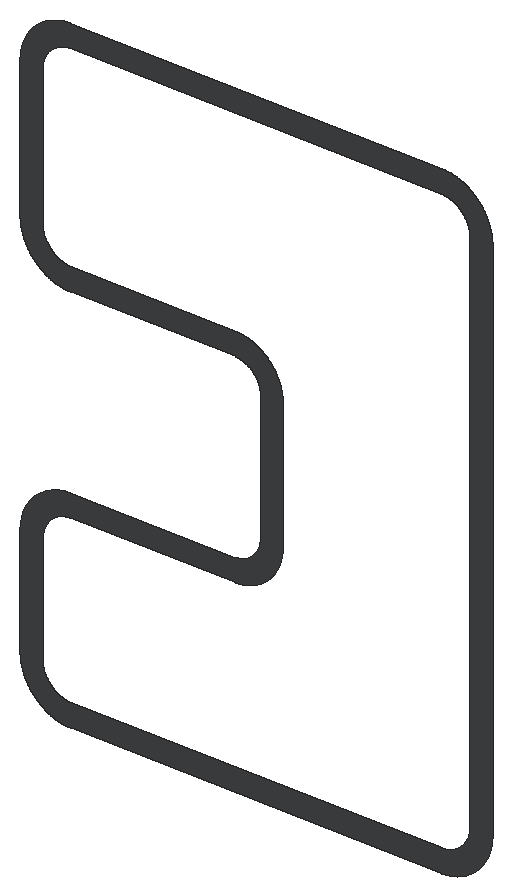
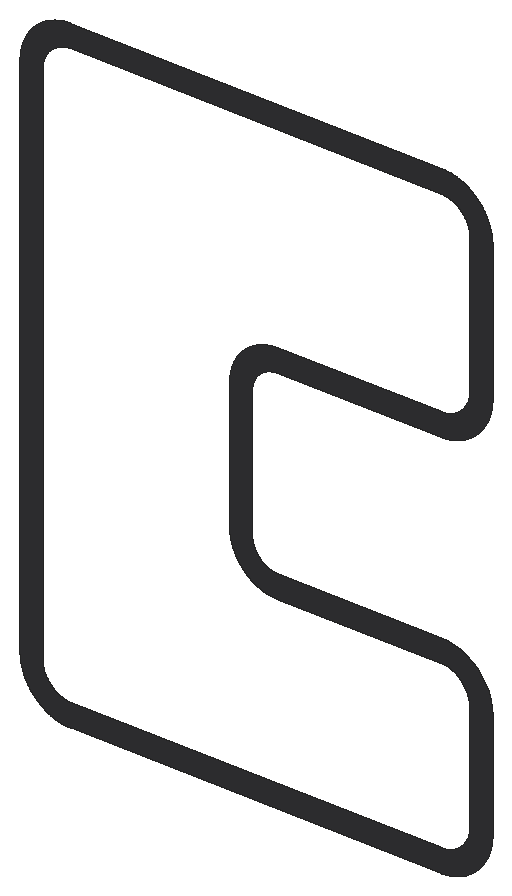
# SketchUp Ruby script. Lengths in inches.
U = 1.inch
M = Sketchup.active_model
def pt(a) = Geom::Point3d.new(a.map { |v| v * U })
def face(e, loops, mat)
  f = e.add_face(loops[0].map { |a| pt(a) })
  loops[1..].each { |l| e.add_face(l.map { |a| pt(a) }).erase! }
  f.material = f.back_material = mat if mat
  f
end
# faces: each face lists its corners as indices into pts; further lists are holes
def faces(e, pts, list, mat = nil) = list.each { |f| face(e, (f[0].is_a?(Array) ? f : [f]).map { |l| l.map { |i| pts[i] } }, mat) }
# xy, xz, yz: faces in a plane at the given z, y or x. An outline is a flat list of corners, or four numbers for a rectangle; further outlines are holes
def ring(l) = l.size == 4 ? [[l[0], l[1]], [l[2], l[1]], [l[2], l[3]], [l[0], l[3]]] : l.each_slice(2).to_a
def flat(e, list, mat, &to3) = list.each { |f| face(e, (f[0].is_a?(Array) ? f : [f]).map { |l| ring(l).map { |u, v| to3.(u, v) } }, mat) }
def xy(e, z, list, mat = nil) = flat(e, list, mat) { |x, y| [x, y, z] }
def xz(e, y, list, mat = nil) = flat(e, list, mat) { |x, z| [x, y, z] }
def yz(e, x, list, mat = nil) = flat(e, list, mat) { |y, z| [x, y, z] }
def lines(e, pts, list) = list.each { |a, b| e.add_line(pt(pts[a]), pt(pts[b])) }
# prism: a flat outline (further loops are holes) pulled along v
def prism(e, loops, v, mat = nil)
  f = face(e, loops, mat); d = Geom::Vector3d.new(v.map { |x| x * U })
  f.pushpull(f.normal.samedirection?(d) ? d.length : -d.length)
end
def box(e, o, s, mat = nil) = prism(e, [[o, [o[0] + s[0], o[1], o[2]], [o[0] + s[0], o[1] + s[1], o[2]], [o[0], o[1] + s[1], o[2]]]], [0, 0, s[2]], mat)
def at(x, y, z, deg = 0) = Geom::Transformation.translation(pt([x, y, z])) * Geom::Transformation.rotation(ORIGIN, Z_AXIS, deg.degrees)
def axes(o, x, y, z) = Geom::Transformation.new([*x, 0, *y, 0, *z, 0, *pt(o).to_a, 1])
def part(name) = M.definitions.add(name)
# library, detail: a bought-in or finely detailed component or shape, given as its bounding box
def library(name, o, s) = part(name).tap { |d| box(d.entities, o, s) }
def detail(e, o, s) = box(e.add_group.entities, o, s)
def put(e, d, t, mat = nil) = e.add_instance(d, t).tap { |i| i.material = mat if mat }
def group(e, t, mat = nil) = e.add_group.tap { |g| g.transformation = t; g.material = mat if mat }.entities
root = M.entities
M.materials.add("1432 AP 8245 TAR ROAD").color = [71, 72, 75]
xz(root,95.37,[[[278.72,155.79,537.28,155.79,537.57,155.8,537.85,155.8,538.41,155.82,538.7,155.83,538.98,155.85,539.26,155.86,539.82,155.9,540.11,155.93,540.39,155.95,541.23,156.04,541.51,156.08,541.79,156.11,542.35,156.19,542.63,156.24,542.91,156.28,543.1875,156.33,543.47,156.38,543.75,156.43,544.02,156.48,544.58,156.6,544.85,156.66,545.13,156.72,545.4,156.79,545.68,156.85,545.95,156.92,546.23,156.99,546.5,157.07,546.77,157.14,547.31,157.3,547.59,157.38,547.86,157.47,548.125,157.55,548.39,157.64,548.66,157.73,548.93,157.83,549.19,157.92,549.73,158.12,550.25,158.32,550.51,158.43,550.78,158.53,551.3,158.75,551.56,158.87,551.81,158.98,552.33,159.22,552.58,159.34,552.84,159.46,553.34,159.72,553.6,159.85,553.85,159.98,554.09,160.11,554.34,160.25,554.59,160.38,554.84,160.52,555.08,160.66,555.33,160.81,555.57,160.95,556.53,161.55,556.76,161.7,557.24,162.02,557.93,162.5,558.16,162.67,558.39,162.83,558.62,163,558.84,163.17,559.06,163.35,559.29,163.52,559.51,163.7,559.95,164.05,560.16,164.23,560.38,164.42,560.59,164.6,560.81,164.79,561.23,165.17,561.4375,165.36,561.64,165.55,561.85,165.74,562.05,165.94,562.26,166.14,562.46,166.34,562.65,166.54,563.05,166.94,563.24,167.15,563.4375,167.36,563.625,167.5625,563.82,167.77,564,167.98,564.19,168.2,564.375,168.41,564.56,168.63,564.74,168.84,564.92,169.0625,565.1,169.28,565.27,169.5,565.45,169.73,565.62,169.95,565.79,170.18,565.96,170.4,566.29,170.86,566.45,171.09,566.62,171.32,566.77,171.56,566.93,171.79,567.09,172.03,567.24,172.26,567.4,172.5,567.7,172.98,567.84,173.22,567.99,173.47,568.13,173.71,568.27,173.96,568.41,174.2,568.55,174.45,568.68,174.7,568.82,174.95,569.08,175.45,569.2,175.7,569.33,175.95,569.45,176.21,569.57,176.46,569.69,176.72,569.8125,176.98,569.93,177.24,570.04,177.49,570.15,177.75,570.26,178.02,570.37,178.28,570.47,178.54,570.58,178.8,570.68,179.07,570.77,179.33,570.87,179.6,570.97,179.86,571.24,180.67,571.32,180.9375,571.41,181.21,571.65,182.02,571.72,182.29,571.8,182.57,571.87,182.84,571.9375,183.11,572.01,183.39,572.07,183.66,572.13,183.9375,572.19,184.22,572.25,184.49,572.31,184.77,572.36,185.05,572.41,185.32,572.56,186.16,572.72,187.28,572.75,187.5625,572.78,187.84,572.8125,188.12,572.84,188.4,572.87,188.6875,572.89,188.97,572.93,189.53,572.95,189.8125,572.96,190.1,572.99,190.94,573,191.23,573,561.36,572.98,561.92,572.97,562.21,572.95,562.77,572.91,563.33,572.89,563.62,572.87,563.9,572.84,564.18,572.8125,564.46,572.78,564.74,572.72,565.3,572.56,566.42,572.31,567.82,572.25,568.09,572.13,568.65,572.07,568.92,572.01,569.2,571.9375,569.47,571.8,570.02,571.72,570.29,571.65,570.5625,571.57,570.84,571.41,571.38,571.32,571.65,571.24,571.92,571.15,572.19,571.06,572.45,570.97,572.72,570.87,572.99,570.77,573.25,570.68,573.52,570.58,573.78,570.47,574.04,570.37,574.31,569.93,575.35,569.8125,575.61,569.69,575.86,569.57,576.12,569.33,576.63,569.2,576.88,569.08,577.14,568.82,577.64,568.68,577.89,568.55,578.14,568.41,578.38,568.27,578.63,567.99,579.12,567.84,579.36,567.7,579.6,567.4,580.08,567.24,580.32,567.09,580.56,566.93,580.79,566.77,581.03,566.62,581.26,566.45,581.49,566.29,581.72,565.96,582.18,565.79,582.41,565.62,582.63,565.45,582.86,565.27,583.08,565.1,583.3,564.56,583.96,564.375,584.17,564.19,584.39,564,584.6,563.82,584.8125,563.625,585.02,563.4375,585.23,563.24,585.4375,563.05,585.64,562.85,585.84,562.65,586.05,562.46,586.25,562.26,586.45,562.05,586.64,561.85,586.84,561.64,587.03,561.4375,587.23,561.23,587.42,560.81,587.8,560.59,587.98,560.38,588.17,560.16,588.35,559.95,588.53,559.51,588.89,559.29,589.0625,559.06,589.24,558.62,589.58,558.16,589.92,557.93,590.08,557.7,590.25,557.24,590.57,557,590.72,556.76,590.88,556.53,591.04,556.29,591.1875,556.05,591.34,555.81,591.49,555.57,591.63,555.33,591.78,555.08,591.92,554.84,592.0625,554.59,592.2,554.34,592.34,554.09,592.47,553.85,592.61,553.6,592.74,553.34,592.87,553.09,593,552.84,593.12,552.58,593.24,552.33,593.37,552.07,593.49,551.81,593.6,551.56,593.72,550.78,594.05,550.51,594.16,550.25,594.26,549.99,594.37,549.73,594.47,549.46,594.57,549.19,594.66,548.93,594.76,548.39,594.94,547.86,595.12,547.59,595.2,547.31,595.28,546.5,595.52,546.23,595.59,545.95,595.66,545.68,595.73,545.4,595.8,545.13,595.86,544.85,595.93,544.58,595.99,544.3,596.04,544.02,596.1,543.75,596.15,543.47,596.21,543.1875,596.26,542.91,596.3,542.63,596.35,541.51,596.51,540.11,596.66,539.82,596.68,538.98,596.74,538.7,596.75,538.41,596.76,537.57,596.79,278.43,596.79,277.59,596.76,277.3,596.75,277.02,596.74,276.18,596.68,275.89,596.66,274.49,596.51,273.37,596.35,273.09,596.3,272.8125,596.26,272.53,596.21,272.25,596.15,271.98,596.1,271.7,596.04,271.42,595.99,271.15,595.93,270.87,595.86,270.6,595.8,270.32,595.73,270.05,595.66,269.77,595.59,269.5,595.52,268.69,595.28,268.41,595.2,268.14,595.12,267.61,594.94,267.07,594.76,266.81,594.66,266.54,594.57,266.27,594.47,266.01,594.37,265.75,594.26,265.49,594.16,265.22,594.05,264.44,593.72,264.19,593.6,263.93,593.49,263.67,593.37,263.42,593.24,263.16,593.12,262.91,593,262.66,592.87,262.4,592.74,262.15,592.61,261.91,592.47,261.66,592.34,261.41,592.2,261.16,592.0625,260.92,591.92,260.67,591.78,260.43,591.63,260.19,591.49,259.95,591.34,259.71,591.1875,259.47,591.04,259.24,590.88,259,590.72,258.76,590.57,258.3,590.25,258.07,590.08,257.84,589.92,257.38,589.58,256.94,589.24,256.71,589.0625,256.49,588.89,256.05,588.53,255.84,588.35,255.62,588.17,255.41,587.98,255.19,587.8,254.77,587.42,254.5625,587.23,254.36,587.03,254.15,586.84,253.95,586.64,253.74,586.45,253.54,586.25,253.35,586.05,253.15,585.84,252.95,585.64,252.76,585.4375,252.5625,585.23,252.375,585.02,252.18,584.8125,252,584.6,251.81,584.39,251.625,584.17,251.44,583.96,250.9,583.3,250.73,583.08,250.55,582.86,250.38,582.63,250.21,582.41,250.04,582.18,249.71,581.72,249.55,581.49,249.38,581.26,249.23,581.03,249.07,580.79,248.91,580.56,248.76,580.32,248.6,580.08,248.3,579.6,248.16,579.36,248.01,579.12,247.73,578.63,247.59,578.38,247.45,578.14,247.32,577.89,247.18,577.64,246.92,577.14,246.8,576.88,246.67,576.63,246.43,576.12,246.31,575.86,246.1875,575.61,246.07,575.35,245.63,574.31,245.53,574.04,245.42,573.78,245.32,573.52,245.23,573.25,245.13,572.99,245.03,572.72,244.94,572.45,244.85,572.19,244.76,571.92,244.68,571.65,244.59,571.38,244.43,570.84,244.35,570.5625,244.28,570.29,244.2,570.02,244.0625,569.47,243.99,569.2,243.93,568.92,243.87,568.65,243.75,568.09,243.69,567.82,243.44,566.42,243.28,565.3,243.22,564.74,243.1875,564.46,243.16,564.18,243.13,563.9,243.11,563.62,243.09,563.33,243.05,562.77,243.03,562.21,243.02,561.92,243,561.36,243,464.23,243.01,463.94,243.04,463.1,243.05,462.8125,243.07,462.53,243.11,461.97,243.13,461.6875,243.16,461.4,243.1875,461.12,243.22,460.84,243.25,460.5625,243.28,460.28,243.44,459.16,243.59,458.32,243.64,458.05,243.69,457.77,243.75,457.49,243.81,457.22,243.87,456.9375,243.93,456.66,243.99,456.39,244.0625,456.11,244.13,455.84,244.2,455.57,244.28,455.29,244.35,455.02,244.59,454.21,244.68,453.9375,244.76,453.67,245.03,452.86,245.13,452.6,245.23,452.33,245.32,452.07,245.42,451.8,245.53,451.54,245.63,451.28,245.74,451.02,245.85,450.75,245.96,450.49,246.07,450.24,246.1875,449.98,246.31,449.72,246.43,449.46,246.55,449.21,246.67,448.95,246.8,448.7,246.92,448.45,247.18,447.95,247.32,447.7,247.45,447.45,247.59,447.2,247.73,446.96,247.87,446.71,248.01,446.47,248.16,446.22,248.3,445.98,248.6,445.5,248.76,445.26,248.91,445.03,249.07,444.79,249.23,444.56,249.38,444.32,249.55,444.09,249.71,443.86,250.04,443.4,250.21,443.18,250.38,442.95,250.55,442.73,250.73,442.5,250.9,442.28,251.08,442.0625,251.26,441.84,251.44,441.63,251.625,441.41,251.81,441.2,252,440.98,252.18,440.77,252.375,440.5625,252.5625,440.36,252.76,440.15,252.95,439.94,253.35,439.54,253.54,439.34,253.74,439.14,253.95,438.94,254.15,438.74,254.36,438.55,254.5625,438.36,254.77,438.17,255.19,437.79,255.41,437.6,255.62,437.42,255.84,437.23,256.05,437.05,256.49,436.7,256.71,436.52,256.94,436.35,257.16,436.17,257.38,436,257.61,435.83,257.84,435.67,258.07,435.5,258.76,435.02,259.24,434.7,259.47,434.55,260.43,433.95,260.67,433.81,260.92,433.66,261.16,433.52,261.41,433.38,261.66,433.25,261.91,433.11,262.15,432.98,262.4,432.85,262.66,432.72,263.16,432.46,263.42,432.34,263.67,432.22,264.19,431.98,264.44,431.87,264.7,431.75,265.22,431.53,265.49,431.43,265.75,431.32,266.27,431.12,266.81,430.92,267.07,430.83,267.34,430.73,267.61,430.64,267.875,430.55,268.14,430.47,268.41,430.38,268.69,430.3,269.23,430.14,269.5,430.07,269.77,429.99,270.05,429.92,270.32,429.85,270.6,429.79,270.87,429.72,271.15,429.66,271.42,429.6,271.98,429.48,272.25,429.43,272.53,429.38,272.8125,429.33,273.09,429.28,273.37,429.24,273.65,429.19,274.21,429.11,274.49,429.08,274.77,429.04,275.61,428.95,275.89,428.93,276.18,428.9,276.74,428.86,277.02,428.85,277.3,428.83,277.59,428.82,278.15,428.8,278.43,428.8,278.72,428.79,393.47,428.79,393.71,428.78,393.94,428.77,394.18,428.75,394.41,428.74,394.65,428.72,394.88,428.69,395.12,428.67,395.58,428.61,395.82,428.57,396.51,428.45,396.97,428.35,397.2,428.29,397.43,428.24,397.89,428.12,398.11,428.05,398.34,427.98,398.5625,427.91,398.79,427.84,399.45,427.6,400.11,427.33,400.32,427.24,400.54,427.14,400.75,427.04,400.96,426.9375,401.17,426.83,401.8,426.5,402.4,426.14,402.61,426.02,402.8,425.89,403,425.76,403.2,425.625,403.39,425.49,403.96,425.07,404.14,424.93,404.33,424.78,404.87,424.33,405.04,424.17,405.22,424.01,405.56,423.69,405.73,423.52,405.89,423.35,406.06,423.18,406.22,423.01,406.375,422.84,406.53,422.66,406.6875,422.48,406.84,422.3,406.99,422.12,407.14,421.9375,407.42,421.5625,407.5625,421.37,407.7,421.18,407.83,420.99,407.97,420.79,408.1,420.6,408.22,420.4,408.35,420.2,408.47,420,408.59,419.79,408.7,419.59,408.82,419.38,409.04,418.96,409.14,418.75,409.25,418.54,409.35,418.33,409.44,418.11,409.54,417.9,409.72,417.46,409.8,417.24,409.89,417.02,409.97,416.8,410.04,416.58,410.12,416.35,410.19,416.13,410.26,415.9,410.32,415.68,410.39,415.45,410.45,415.22,410.5,414.99,410.56,414.76,410.61,414.53,410.65,414.3,410.7,414.07,410.78,413.61,410.8125,413.375,410.85,413.14,410.875,412.91,410.9,412.67,410.92,412.4375,410.94,412.2,410.96,411.97,410.98,411.73,410.99,411.5,410.99,411.26,411,411.03,411,320.56,410.99,320.32,410.99,320.09,410.98,319.85,410.96,319.61,410.92,319.15,410.9,318.91,410.875,318.68,410.85,318.44,410.8125,318.21,410.78,317.98,410.74,317.74,410.7,317.51,410.65,317.28,410.61,317.05,410.56,316.82,410.5,316.59,410.45,316.36,410.39,316.13,410.32,315.91,410.26,315.68,410.19,315.45,410.12,315.23,410.04,315.01,409.97,314.78,409.89,314.5625,409.8,314.34,409.72,314.12,409.63,313.9,409.54,313.6875,409.44,313.47,409.35,313.26,409.25,313.04,409.14,312.83,409.04,312.62,408.82,312.2,408.7,312,408.59,311.79,408.35,311.39,408.22,311.1875,408.1,310.99,407.97,310.79,407.83,310.6,407.7,310.4,407.5625,310.21,407.42,310.02,407.28,309.83,407.14,309.65,406.99,309.46,406.84,309.28,406.6875,309.1,406.53,308.92,406.375,308.75,406.22,308.57,406.06,308.4,405.89,308.23,405.73,308.0625,405.56,307.9,405.39,307.74,405.22,307.57,405.04,307.42,404.87,307.26,404.69,307.1,404.33,306.8,404.14,306.66,403.96,306.51,403.39,306.09,403.2,305.96,402.8,305.7,402.61,305.57,402.4,305.44,402,305.2,401.8,305.09,401.59,304.97,401.17,304.75,400.54,304.45,400.32,304.35,400.11,304.25,399.67,304.07,399.45,303.99,399.23,303.9,399.01,303.82,398.79,303.75,398.5625,303.67,398.34,303.6,398.11,303.53,397.89,303.47,397.2,303.29,396.28,303.09,395.82,303.01,395.58,302.98,395.12,302.92,394.88,302.89,394.65,302.87,394.41,302.85,394.18,302.83,393.94,302.82,393.71,302.81,393.47,302.8,393.24,302.79,279,302.79,274.3,302.48,269.68,301.57,265.22,300.05,261,297.97,257.08,295.35,253.54,292.25,250.4375,288.71,247.82,284.79,245.74,280.57,244.23,276.11,243.31,271.49,243,266.79,243,191.23,243.01,190.94,243.04,190.1,243.05,189.8125,243.07,189.53,243.11,188.97,243.13,188.6875,243.16,188.4,243.1875,188.12,243.22,187.84,243.25,187.5625,243.28,187.28,243.44,186.16,243.59,185.32,243.64,185.05,243.69,184.77,243.75,184.49,243.81,184.22,243.87,183.9375,243.93,183.66,243.99,183.39,244.0625,183.11,244.13,182.84,244.2,182.57,244.28,182.29,244.35,182.02,244.59,181.21,244.68,180.9375,244.76,180.67,245.03,179.86,245.13,179.6,245.23,179.33,245.32,179.07,245.42,178.8,245.53,178.54,245.63,178.28,245.74,178.02,245.85,177.75,245.96,177.49,246.07,177.24,246.1875,176.98,246.31,176.72,246.43,176.46,246.55,176.21,246.67,175.95,246.8,175.7,246.92,175.45,247.18,174.95,247.32,174.7,247.45,174.45,247.59,174.2,247.73,173.96,247.87,173.71,248.01,173.47,248.16,173.22,248.3,172.98,248.6,172.5,248.76,172.26,248.91,172.03,249.07,171.79,249.23,171.56,249.38,171.32,249.55,171.09,249.71,170.86,250.04,170.4,250.21,170.18,250.38,169.95,250.55,169.73,250.73,169.5,250.9,169.28,251.08,169.0625,251.26,168.84,251.44,168.63,251.625,168.41,251.81,168.2,252,167.98,252.18,167.77,252.375,167.5625,252.5625,167.36,252.76,167.15,252.95,166.94,253.35,166.54,253.54,166.34,253.74,166.14,253.95,165.94,254.15,165.74,254.36,165.55,254.5625,165.36,254.77,165.17,255.19,164.79,255.41,164.6,255.62,164.42,255.84,164.23,256.05,164.05,256.49,163.7,256.71,163.52,256.94,163.35,257.16,163.17,257.38,163,257.61,162.83,257.84,162.67,258.07,162.5,258.76,162.02,259.24,161.7,259.47,161.55,260.43,160.95,260.67,160.81,260.92,160.66,261.16,160.52,261.41,160.38,261.66,160.25,261.91,160.11,262.15,159.98,262.4,159.85,262.66,159.72,263.16,159.46,263.42,159.34,263.67,159.22,264.19,158.98,264.44,158.87,264.7,158.75,265.22,158.53,265.49,158.43,265.75,158.32,266.27,158.12,266.81,157.92,267.07,157.83,267.34,157.73,267.61,157.64,267.875,157.55,268.14,157.47,268.41,157.38,268.69,157.3,269.23,157.14,269.5,157.07,269.77,156.99,270.05,156.92,270.32,156.85,270.6,156.79,270.87,156.72,271.15,156.66,271.42,156.6,271.98,156.48,272.25,156.43,272.53,156.38,272.8125,156.33,273.09,156.28,273.37,156.24,273.65,156.19,274.21,156.11,274.49,156.08,274.77,156.04,275.61,155.95,275.89,155.93,276.18,155.9,276.74,155.86,277.02,155.85,277.3,155.83,277.59,155.82,278.15,155.8,278.43,155.8],[278.68,171.29,278.52,171.3,278.36,171.3,278.2,171.31,278.03,171.31,277.875,171.32,277.71,171.33,277.55,171.34,277.39,171.36,277.07,171.38,276.75,171.42,276.59,171.43,276.27,171.47,276.11,171.5,275.79,171.54,275.63,171.57,275.48,171.6,275.32,171.625,275.16,171.66,275,171.6875,274.84,171.72,274.69,171.75,274.53,171.79,274.37,171.82,274.21,171.86,274.06,171.9,273.9,171.9375,273.75,171.98,273.59,172.02,273.44,172.0625,273.28,172.11,273.125,172.15,272.97,172.2,272.67,172.3,272.51,172.35,272.06,172.5,271.9,172.56,271.75,172.62,271.6,172.67,271.15,172.85,271.01,172.91,270.86,172.98,270.71,173.04,270.5625,173.11,270.42,173.18,270.27,173.24,270.125,173.3125,269.98,173.38,269.84,173.45,269.69,173.53,269.41,173.67,269.27,173.75,268.98,173.91,268.56,174.15,268.43,174.23,268.29,174.3125,268.15,174.4,268.02,174.48,267.88,174.57,267.75,174.66,267.61,174.75,267.48,174.84,267.34,174.93,267.08,175.11,266.95,175.21,266.82,175.3,266.69,175.4,266.5625,175.5,266.44,175.59,266.18,175.79,266.06,175.89,265.93,176,265.81,176.1,265.6875,176.2,265.5625,176.31,265.44,176.41,265.08,176.74,264.97,176.85,264.73,177.07,264.39,177.41,264.28,177.53,264.17,177.64,264.06,177.76,263.95,177.875,263.84,178,263.73,178.11,263.62,178.24,263.52,178.36,263.41,178.48,263.31,178.6,263.2,178.72,263.1,178.85,263,178.97,262.7,179.36,262.61,179.48,262.51,179.61,262.42,179.74,262.32,179.875,262.23,180,262.14,180.14,262.04,180.27,261.95,180.4,261.87,180.54,261.78,180.67,261.69,180.81,261.61,180.94,261.52,181.08,261.4375,181.22,261.35,181.36,261.11,181.78,261.04,181.92,260.88,182.2,260.81,182.34,260.73,182.49,260.59,182.77,260.52,182.92,260.45,183.0625,260.38,183.21,260.32,183.36,260.25,183.5,260.1875,183.65,260.12,183.8,259.82,184.55,259.77,184.7,259.71,184.85,259.61,185.15,259.55,185.3,259.5,185.46,259.45,185.61,259.41,185.76,259.36,185.92,259.3125,186.07,259.27,186.23,259.23,186.38,259.18,186.54,259.14,186.69,259.1,186.85,259.07,187.01,259.03,187.16,258.99,187.32,258.96,187.48,258.93,187.63,258.89,187.79,258.83,188.11,258.81,188.27,258.75,188.59,258.73,188.74,258.7,188.9,258.68,189.0625,258.66,189.22,258.64,189.38,258.61,189.7,258.59,189.86,258.58,190.02,258.5625,190.18,258.55,190.34,258.54,190.5,258.53,190.67,258.52,190.83,258.52,190.99,258.51,191.15,258.51,191.31,258.5,191.47,258.5,266.79,258.68,269.47,259.2,272.1,260.06,274.64,261.25,277.04,262.74,279.27,264.5,281.29,266.52,283.06,268.75,284.55,271.15,285.73,273.69,286.59,276.32,287.12,279,287.29,393.4375,287.29,393.875,287.3,394.32,287.32,394.75,287.34,395.19,287.36,395.63,287.4,396.07,287.43,396.5,287.48,396.9375,287.52,397.37,287.58,397.81,287.64,398.24,287.7,398.67,287.78,399.1,287.85,399.54,287.9375,399.97,288.02,400.39,288.12,401.25,288.32,401.67,288.43,402.51,288.67,403.35,288.93,403.77,289.07,404.18,289.21,404.59,289.36,405.01,289.52,405.41,289.68,405.82,289.84,406.22,290.01,406.625,290.1875,407.03,290.37,407.42,290.56,407.82,290.75,408.21,290.94,408.6,291.14,408.98,291.35,409.37,291.5625,409.75,291.78,410.13,292,410.5,292.23,410.875,292.46,411.25,292.7,411.61,292.9375,411.97,293.18,412.33,293.43,412.69,293.69,413.39,294.21,413.74,294.48,414.76,295.32,415.42,295.9,415.74,296.19,416.06,296.49,416.375,296.8,416.6875,297.1,417,297.42,417.3,297.73,417.6,298.05,417.9,298.375,418.1875,298.7,418.47,299.04,418.76,299.37,419.03,299.71,419.31,300.05,419.58,300.4,420.1,301.1,420.36,301.46,420.61,301.82,420.85,302.18,421.1,302.55,421.33,302.92,421.5625,303.29,421.79,303.66,422.23,304.42,422.44,304.81,422.65,305.19,422.85,305.58,423.05,305.98,423.24,306.37,423.78,307.57,423.95,307.97,424.12,308.38,424.27,308.79,424.43,309.2,424.58,309.61,424.72,310.02,424.86,310.44,425.12,311.28,425.36,312.12,425.47,312.55,425.57,312.97,425.77,313.83,425.86,314.26,425.9375,314.6875,426.02,315.12,426.09,315.55,426.15,315.99,426.27,316.85,426.32,317.29,426.36,317.73,426.4,318.16,426.43,318.6,426.49,319.92,426.5,320.35,426.5,411.23,426.49,411.67,426.45,412.55,426.43,412.98,426.4,413.42,426.36,413.86,426.32,414.29,426.27,414.73,426.21,415.16,426.15,415.6,426.09,416.03,426.02,416.47,425.9375,416.9,425.86,417.33,425.77,417.76,425.67,418.19,425.57,418.61,425.47,419.04,425.36,419.46,425.24,419.89,425.12,420.31,424.99,420.73,424.86,421.14,424.72,421.56,424.58,421.97,424.43,422.39,424.27,422.8,424.12,423.21,423.95,423.61,423.78,424.02,423.42,424.82,423.24,425.21,423.05,425.61,422.65,426.39,422.44,426.78,422.23,427.16,421.79,427.92,421.5625,428.3,421.33,428.67,421.1,429.04,420.85,429.4,420.61,429.77,420.36,430.125,420.1,430.48,419.84,430.84,419.58,431.1875,419.31,431.53,419.03,431.875,418.76,432.21,418.47,432.55,418.1875,432.88,417.9,433.21,417,434.17,416.375,434.79,416.06,435.09,415.74,435.39,415.42,435.6875,415.09,435.98,414.76,436.27,414.08,436.83,413.74,437.1,413.39,437.37,412.69,437.89,412.33,438.15,411.61,438.65,411.25,438.89,410.5,439.36,410.13,439.58,409.37,440.02,408.98,440.23,408.6,440.4375,408.21,440.64,407.82,440.84,407.42,441.03,407.03,441.21,406.625,441.4,406.22,441.57,405.82,441.74,405.41,441.91,405.01,442.07,404.59,442.22,404.18,442.37,403.77,442.51,402.93,442.79,401.67,443.15,401.25,443.26,400.82,443.37,400.39,443.47,399.97,443.56,399.54,443.65,399.1,443.73,398.67,443.81,397.81,443.95,397.37,444.01,396.9375,444.06,396.5,444.11,396.07,444.15,395.63,444.1875,395.19,444.22,394.75,444.25,394.32,444.27,393.875,444.28,393.4375,444.29,278.68,444.29,278.52,444.3,278.36,444.3,278.2,444.31,278.03,444.31,277.875,444.32,277.71,444.33,277.55,444.34,277.39,444.36,277.07,444.38,276.75,444.42,276.59,444.43,276.27,444.47,276.11,444.5,275.79,444.54,275.63,444.57,275.48,444.6,275.32,444.625,275.16,444.66,275,444.6875,274.84,444.72,274.69,444.75,274.53,444.79,274.37,444.82,274.21,444.86,274.06,444.9,273.9,444.9375,273.75,444.98,273.59,445.02,273.44,445.0625,273.28,445.11,273.125,445.15,272.97,445.2,272.67,445.3,272.51,445.35,272.06,445.5,271.9,445.56,271.75,445.62,271.6,445.67,271.15,445.85,271.01,445.91,270.86,445.98,270.71,446.04,270.5625,446.11,270.42,446.18,270.27,446.24,270.125,446.3125,269.98,446.38,269.84,446.45,269.69,446.53,269.41,446.67,269.27,446.75,268.98,446.91,268.56,447.15,268.43,447.23,268.29,447.3125,268.15,447.4,268.02,447.48,267.88,447.57,267.75,447.66,267.61,447.75,267.48,447.84,267.34,447.93,267.08,448.11,266.95,448.21,266.82,448.3,266.69,448.4,266.5625,448.5,266.44,448.59,266.18,448.79,266.06,448.89,265.93,449,265.81,449.1,265.6875,449.2,265.5625,449.31,265.44,449.41,265.08,449.74,264.97,449.85,264.73,450.07,264.39,450.41,264.28,450.53,264.17,450.64,264.06,450.76,263.95,450.875,263.84,451,263.73,451.11,263.62,451.24,263.52,451.36,263.41,451.48,263.31,451.6,263.2,451.72,263.1,451.85,263,451.97,262.7,452.36,262.61,452.48,262.51,452.61,262.42,452.74,262.32,452.875,262.23,453,262.14,453.14,262.04,453.27,261.95,453.4,261.87,453.54,261.78,453.67,261.69,453.81,261.61,453.94,261.52,454.08,261.4375,454.22,261.35,454.36,261.11,454.78,261.04,454.92,260.88,455.2,260.81,455.34,260.73,455.49,260.59,455.77,260.52,455.92,260.45,456.0625,260.38,456.21,260.32,456.36,260.25,456.5,260.1875,456.65,260.12,456.8,259.82,457.55,259.77,457.7,259.71,457.85,259.61,458.15,259.55,458.3,259.5,458.46,259.45,458.61,259.41,458.76,259.36,458.92,259.3125,459.07,259.27,459.23,259.23,459.38,259.18,459.54,259.14,459.69,259.1,459.85,259.07,460.01,259.03,460.16,258.99,460.32,258.96,460.48,258.93,460.63,258.89,460.79,258.83,461.11,258.81,461.27,258.75,461.59,258.73,461.74,258.7,461.9,258.68,462.0625,258.66,462.22,258.64,462.38,258.61,462.7,258.59,462.86,258.58,463.02,258.5625,463.18,258.55,463.34,258.54,463.5,258.53,463.67,258.52,463.83,258.52,463.99,258.51,464.15,258.51,464.31,258.5,464.47,258.5,561.11,258.51,561.28,258.51,561.4375,258.52,561.6,258.52,561.76,258.55,562.24,258.5625,562.4,258.58,562.5625,258.59,562.72,258.61,562.88,258.64,563.2,258.7,563.68,258.73,563.84,258.75,564,258.81,564.32,258.83,564.48,258.86,564.63,258.89,564.79,258.93,564.95,258.96,565.11,258.99,565.26,259.07,565.58,259.1,565.73,259.18,566.05,259.23,566.2,259.27,566.36,259.3125,566.51,259.36,566.67,259.41,566.82,259.45,566.97,259.55,567.28,259.61,567.43,259.66,567.58,259.71,567.74,259.77,567.89,259.82,568.04,259.88,568.1875,259.94,568.34,260.12,568.79,260.1875,568.93,260.25,569.08,260.32,569.23,260.38,569.375,260.45,569.52,260.52,569.67,260.59,569.8125,260.66,569.96,260.73,570.1,260.81,570.24,260.88,570.38,260.96,570.53,261.04,570.67,261.11,570.81,261.35,571.23,261.4375,571.37,261.52,571.5,261.61,571.64,261.69,571.78,261.78,571.91,261.87,572.05,261.95,572.18,262.04,572.31,262.14,572.45,262.32,572.71,262.42,572.84,262.51,572.97,262.61,573.1,262.7,573.23,262.8,573.36,262.9,573.48,263,573.61,263.1,573.73,263.2,573.86,263.31,573.98,263.41,574.11,263.52,574.23,263.62,574.35,264.06,574.83,264.17,574.94,264.28,575.06,264.39,575.17,264.5,575.29,264.62,575.4,264.73,575.51,264.97,575.74,265.08,575.85,265.2,575.95,265.32,576.0625,265.44,576.17,265.5625,576.28,265.6875,576.38,265.81,576.48,265.93,576.59,266.06,576.69,266.18,576.79,266.44,576.99,266.5625,577.09,266.69,577.1875,266.82,577.28,267.08,577.47,267.21,577.5625,267.34,577.66,267.48,577.75,267.61,577.84,267.75,577.93,267.88,578.01,268.02,578.1,268.15,578.1875,268.29,578.27,268.43,578.35,268.56,578.4375,268.7,578.52,268.98,578.68,269.125,578.76,269.27,578.83,269.41,578.91,269.55,578.98,269.69,579.06,269.84,579.13,269.98,579.2,270.27,579.34,270.42,579.41,270.5625,579.48,270.71,579.54,270.86,579.61,271.01,579.67,271.15,579.73,271.75,579.97,271.9,580.02,272.06,580.08,272.21,580.13,272.36,580.1875,272.51,580.24,272.67,580.29,272.97,580.39,273.125,580.43,273.28,580.48,273.44,580.52,273.59,580.57,273.75,580.61,273.9,580.65,274.06,580.6875,274.21,580.73,274.37,580.76,274.53,580.8,274.69,580.83,274.84,580.87,275.48,580.99,275.63,581.01,275.79,581.04,275.95,581.0625,276.11,581.09,276.91,581.19,277.07,581.2,277.23,581.22,277.71,581.25,277.875,581.26,278.03,581.27,278.2,581.28,278.36,581.28,278.52,581.29,537.48,581.29,537.64,581.28,537.8,581.28,537.97,581.27,538.125,581.26,538.29,581.25,538.77,581.22,538.93,581.2,539.09,581.19,539.89,581.09,540.05,581.0625,540.21,581.04,540.37,581.01,540.52,580.99,541.16,580.87,541.31,580.83,541.47,580.8,541.63,580.76,541.79,580.73,541.94,580.6875,542.1,580.65,542.25,580.61,542.41,580.57,542.56,580.52,542.72,580.48,542.875,580.43,543.03,580.39,543.33,580.29,543.49,580.24,543.64,580.1875,543.79,580.13,543.94,580.08,544.1,580.02,544.25,579.97,544.85,579.73,544.99,579.67,545.14,579.61,545.29,579.54,545.4375,579.48,545.58,579.41,545.73,579.34,546.02,579.2,546.16,579.13,546.31,579.06,546.45,578.98,546.59,578.91,546.73,578.83,546.875,578.76,547.02,578.68,547.3,578.52,547.44,578.4375,547.57,578.35,547.71,578.27,547.85,578.1875,547.98,578.1,548.12,578.01,548.25,577.93,548.39,577.84,548.52,577.75,548.66,577.66,548.79,577.5625,548.92,577.47,549.18,577.28,549.31,577.1875,549.4375,577.09,549.56,576.99,549.82,576.79,549.94,576.69,550.07,576.59,550.19,576.48,550.3125,576.38,550.4375,576.28,550.56,576.17,550.68,576.0625,550.8,575.95,550.92,575.85,551.03,575.74,551.27,575.51,551.38,575.4,551.5,575.29,551.61,575.17,551.72,575.06,551.83,574.94,551.94,574.83,552.38,574.35,552.48,574.23,552.59,574.11,552.69,573.98,552.8,573.86,552.9,573.73,553,573.61,553.1,573.48,553.2,573.36,553.3,573.23,553.39,573.1,553.49,572.97,553.58,572.84,553.68,572.71,553.86,572.45,553.96,572.31,554.05,572.18,554.13,572.05,554.22,571.91,554.31,571.78,554.39,571.64,554.48,571.5,554.5625,571.37,554.65,571.23,554.89,570.81,554.96,570.67,555.04,570.53,555.12,570.38,555.19,570.24,555.27,570.1,555.34,569.96,555.41,569.8125,555.48,569.67,555.55,569.52,555.62,569.375,555.68,569.23,555.75,569.08,555.8125,568.93,555.88,568.79,556.06,568.34,556.12,568.1875,556.18,568.04,556.23,567.89,556.29,567.74,556.34,567.58,556.39,567.43,556.45,567.28,556.55,566.97,556.59,566.82,556.64,566.67,556.6875,566.51,556.73,566.36,556.77,566.2,556.82,566.05,556.9,565.73,556.93,565.58,557.01,565.26,557.04,565.11,557.07,564.95,557.11,564.79,557.14,564.63,557.17,564.48,557.19,564.32,557.25,564,557.27,563.84,557.3,563.68,557.36,563.2,557.39,562.88,557.41,562.72,557.42,562.5625,557.4375,562.4,557.45,562.24,557.48,561.76,557.48,561.6,557.49,561.4375,557.49,561.28,557.5,561.11,557.5,191.47,557.49,191.31,557.49,191.15,557.48,190.99,557.48,190.83,557.47,190.67,557.46,190.5,557.45,190.34,557.4375,190.18,557.42,190.02,557.41,189.86,557.39,189.7,557.36,189.38,557.34,189.22,557.32,189.0625,557.3,188.9,557.27,188.74,557.25,188.59,557.19,188.27,557.17,188.11,557.11,187.79,557.07,187.63,557.04,187.48,557.01,187.32,556.97,187.16,556.93,187.01,556.9,186.85,556.86,186.69,556.82,186.54,556.77,186.38,556.73,186.23,556.6875,186.07,556.64,185.92,556.59,185.76,556.55,185.61,556.5,185.46,556.45,185.3,556.39,185.15,556.29,184.85,556.23,184.7,556.18,184.55,555.88,183.8,555.8125,183.65,555.75,183.5,555.68,183.36,555.62,183.21,555.55,183.0625,555.48,182.92,555.41,182.77,555.27,182.49,555.19,182.34,555.12,182.2,554.96,181.92,554.89,181.78,554.65,181.36,554.5625,181.22,554.48,181.08,554.39,180.94,554.31,180.81,554.22,180.67,554.13,180.54,554.05,180.4,553.96,180.27,553.86,180.14,553.77,180,553.68,179.875,553.58,179.74,553.49,179.61,553.39,179.48,553.3,179.36,553,178.97,552.9,178.85,552.8,178.72,552.69,178.6,552.59,178.48,552.48,178.36,552.38,178.24,552.27,178.11,552.16,178,552.05,177.875,551.94,177.76,551.83,177.64,551.72,177.53,551.61,177.41,551.27,177.07,551.03,176.85,550.92,176.74,550.56,176.41,550.4375,176.31,550.3125,176.2,550.19,176.1,550.07,176,549.94,175.89,549.82,175.79,549.56,175.59,549.4375,175.5,549.31,175.4,549.18,175.3,549.05,175.21,548.92,175.11,548.66,174.93,548.52,174.84,548.39,174.75,548.25,174.66,548.12,174.57,547.98,174.48,547.85,174.4,547.71,174.3125,547.57,174.23,547.44,174.15,547.02,173.91,546.73,173.75,546.59,173.67,546.31,173.53,546.16,173.45,546.02,173.38,545.875,173.3125,545.73,173.24,545.58,173.18,545.4375,173.11,545.29,173.04,545.14,172.98,544.99,172.91,544.85,172.85,544.4,172.67,544.25,172.62,544.1,172.56,543.94,172.5,543.49,172.35,543.33,172.3,543.03,172.2,542.875,172.15,542.72,172.11,542.56,172.0625,542.41,172.02,542.25,171.98,542.1,171.9375,541.94,171.9,541.79,171.86,541.63,171.82,541.47,171.79,541.31,171.75,541.16,171.72,541,171.6875,540.84,171.66,540.68,171.625,540.52,171.6,540.37,171.57,540.21,171.54,539.89,171.5,539.73,171.47,539.41,171.43,539.25,171.42,538.93,171.38,538.61,171.36,538.45,171.34,538.29,171.33,538.125,171.32,537.97,171.31,537.8,171.31,537.64,171.3,537.48,171.3,537.32,171.29]]],"1432 AP 8245 TAR ROAD")
